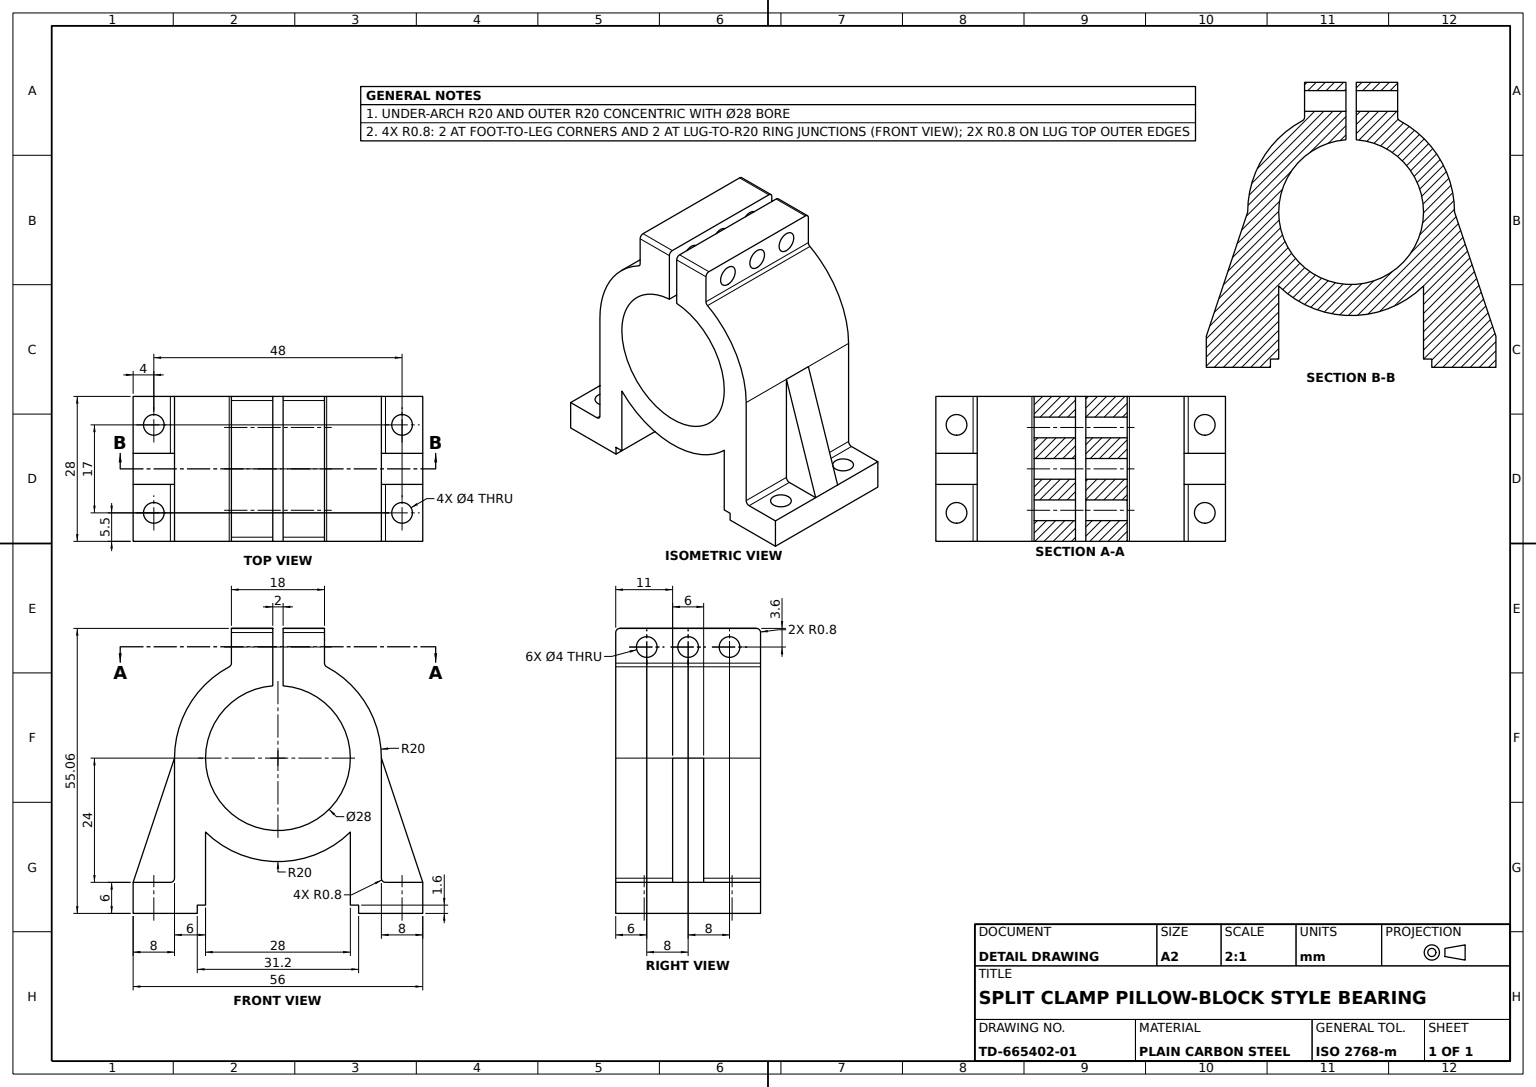
solid
v1 (-28,-24,-11)
v2 (-20.8,-24,-11)
e1 v1 v2 LINE
v3 (-28,-24,0)
e2 v1 v3 LINE
v4 (-20.8,-24,0)
e3 v4 v3 LINE
e4 v4 v2 LINE
v5 (-24,-24,-3.5)
v6 (-24,-24,-7.5)
e5 v5 v6 CIRCLE(AX(P(-24,-24,-5.5),D(0,1,0),D(0,0,1)),2)
e6 v6 v5 CIRCLE(AX(P(-24,-24,-5.5),D(0,1,0),D(0,0,1)),2)
face PLANE(AX(P(-20,-24,-28),D(0,1,0),D(0,0,1))) [-e1 e2 -e3 e4] [-e5 -e6]
v7 (-20,-23.2,-11)
v8 (-20,0,-11)
e7 v7 v8 LINE
e8 v8 v1 LINE
e9 v2 v7 CIRCLE(AX(P(-20.8,-23.2,-11),D(0,0,1),D(1,0,0)),0.8)
face PLANE(AX(P(0,-5,-11),D(0,0,1),D(1,0,0))) [e7 e8 e1 e9]
v9 (-1,23.460571,-22)
v10 (-1,19.460571,-22)
e10 v9 v10 CIRCLE(AX(P(-1,21.460571,-22),D(-1,0,0),D(0,0,1)),2)
v11 (-9,23.460571,-22)
e11 v11 v9 LINE
v12 (-9,19.460571,-22)
e12 v11 v12 CIRCLE(AX(P(-9,21.460571,-22),D(-1,0,0),D(0,0,1)),2)
e13 v12 v10 LINE
face CYL(AX(P(-19,21.460571,-22),D(1,0,0),D(0,1,0)),2) rev [-e10 -e11 e12 e13]
v13 (1,23.460571,-6)
v14 (1,19.460571,-6)
e14 v13 v14 CIRCLE(AX(P(1,21.460571,-6),D(1,0,0),D(0,0,-1)),2)
e15 v14 v13 CIRCLE(AX(P(1,21.460571,-6),D(1,0,0),D(0,0,-1)),2)
v15 (1,25.060571,-0.8)
v16 (1,25.060571,-27.2)
e16 v15 v16 LINE
v17 (1,24.260571,-28)
e17 v16 v17 CIRCLE(AX(P(1,24.260571,-27.2),D(-1,0,0),D(0,0,-1)),0.8)
v18 (1,13.96424,-28)
e18 v18 v17 LINE
v19 (1,13.96424,0)
e19 v19 v18 LINE
v20 (1,24.260571,0)
e20 v19 v20 LINE
e21 v20 v15 CIRCLE(AX(P(1,24.260571,-0.8),D(-1,0,0),D(0,0,-1)),0.8)
v21 (1,23.460571,-14)
v22 (1,19.460571,-14)
e22 v21 v22 CIRCLE(AX(P(1,21.460571,-14),D(1,0,0),D(0,0,-1)),2)
e23 v22 v21 CIRCLE(AX(P(1,21.460571,-14),D(1,0,0),D(0,0,-1)),2)
v23 (1,23.460571,-22)
v24 (1,19.460571,-22)
e24 v23 v24 CIRCLE(AX(P(1,21.460571,-22),D(1,0,0),D(0,0,-1)),2)
e25 v24 v23 CIRCLE(AX(P(1,21.460571,-22),D(1,0,0),D(0,0,-1)),2)
face PLANE(AX(P(1,11.884737,-28),D(1,0,0),D(0,0,-1))) rev [e14 e15] [e16 e17 -e18 -e19 e20 e21] [e22 e23] [e24 e25]
v25 (9,19.460571,-22)
e26 v24 v25 LINE
v26 (9,23.460571,-22)
e27 v23 v26 LINE
e28 v26 v25 CIRCLE(AX(P(9,21.460571,-22),D(1,0,0),D(0,1,0)),2)
face CYL(AX(P(-19,21.460571,-22),D(1,0,0),D(0,1,0)),2) rev [-e26 -e24 e27 e28]
v27 (-9.423077,17.641021,-28)
v28 (-9,18.346662,-28)
e29 v27 v28 CIRCLE(AX(P(-9.8,18.346662,-28),D(0,0,1),D(1,0,0)),0.8)
v29 (-9.423077,17.641021,0)
e30 v29 v27 LINE
v30 (-9,18.346662,0)
e31 v30 v29 CIRCLE(AX(P(-9.8,18.346662,0),D(0,0,-1),D(1,0,0)),0.8)
e32 v28 v30 LINE
face CYL(AX(P(-9.8,18.346662,-28),D(0,0,1),D(1,0,0)),0.8) rev [-e29 -e30 -e31 -e32]
v31 (-9,23.460571,-14)
v32 (-9,19.460571,-14)
e33 v31 v32 CIRCLE(AX(P(-9,21.460571,-14),D(-1,0,0),D(0,0,1)),2)
v33 (-1,19.460571,-14)
e34 v32 v33 LINE
v34 (-1,23.460571,-14)
e35 v34 v33 CIRCLE(AX(P(-1,21.460571,-14),D(-1,0,0),D(0,0,1)),2)
e36 v31 v34 LINE
face CYL(AX(P(-19,21.460571,-14),D(1,0,0),D(0,1,0)),2) rev [e33 e34 -e35 -e36]
v35 (20,0,-11)
v36 (28,-24,-11)
e37 v35 v36 LINE
v37 (28,-24,-17)
e38 v37 v36 LINE
v38 (20,0,-17)
e39 v38 v37 LINE
e40 v38 v35 LINE
face PLANE(AX(P(20,0,-14),D(-0.948683298,-0.316227766,0),D(0.316227766,-0.948683298,0))) rev [e37 -e38 -e39 e40]
v39 (-1,24.260571,-28)
v40 (-1,13.96424,-28)
e41 v39 v40 LINE
v41 (-1,25.060571,-27.2)
e42 v39 v41 CIRCLE(AX(P(-1,24.260571,-27.2),D(1,0,0),D(0,0,1)),0.8)
v42 (-1,25.060571,-0.8)
e43 v41 v42 LINE
v43 (-1,24.260571,0)
e44 v42 v43 CIRCLE(AX(P(-1,24.260571,-0.8),D(1,0,0),D(0,0,1)),0.8)
v44 (-1,13.96424,0)
e45 v43 v44 LINE
e46 v40 v44 LINE
e47 v10 v9 CIRCLE(AX(P(-1,21.460571,-22),D(-1,0,0),D(0,0,1)),2)
e48 v33 v34 CIRCLE(AX(P(-1,21.460571,-14),D(-1,0,0),D(0,0,1)),2)
v45 (-1,23.460571,-6)
v46 (-1,19.460571,-6)
e49 v45 v46 CIRCLE(AX(P(-1,21.460571,-6),D(-1,0,0),D(0,0,1)),2)
e50 v46 v45 CIRCLE(AX(P(-1,21.460571,-6),D(-1,0,0),D(0,0,1)),2)
face PLANE(AX(P(-1,11.884737,-28),D(-1,0,0),D(0,0,1))) rev [-e41 e42 e43 e44 e45 -e46] [e10 e47] [e35 e48] [e49 e50]
v47 (28,-30,-28)
v48 (28,-30,0)
e51 v47 v48 LINE
v49 (28,-24,-28)
e52 v47 v49 LINE
e53 v49 v37 LINE
v50 (28,-24,0)
e54 v36 v50 LINE
e55 v48 v50 LINE
face PLANE(AX(P(28,-24,-28),D(1,0,0),D(0,0,-1))) [-e51 e52 e53 e38 e54 -e55]
v51 (-14,0,0)
e56 v44 v51 CIRCLE(AX(P(0,0,0),D(0,0,1),D(1,0,0)),14)
v52 (-14,0,-28)
e57 v52 v51 LINE
e58 v40 v52 CIRCLE(AX(P(0,0,-28),D(0,0,1),D(1,0,0)),14)
face CYL(AX(P(0,0,-28),D(0,0,1),D(1,0,0)),14) rev [e56 -e57 -e58 e46]
v53 (24,-30,-24.5)
v54 (24,-24,-24.5)
e59 v53 v54 LINE
v55 (24,-30,-20.5)
e60 v53 v55 CIRCLE(AX(P(24,-30,-22.5),D(0,-1,0),D(0,0,-1)),2)
v56 (24,-24,-20.5)
e61 v55 v56 LINE
e62 v56 v54 CIRCLE(AX(P(24,-24,-22.5),D(0,1,0),D(0,0,1)),2)
face CYL(AX(P(24,-52,-22.5),D(0,1,0),D(0,0,1)),2) rev [-e59 e60 e61 e62]
v57 (9,25.060571,-27.2)
v58 (9,25.060571,-0.8)
e63 v57 v58 LINE
e64 v57 v16 LINE
e65 v15 v58 LINE
face PLANE(AX(P(-9,25.060571,-28),D(0,1,0),D(0,0,1))) [-e63 e64 -e16 e65]
v59 (-20,-23.2,-17)
v60 (-20,0,-17)
e66 v59 v60 LINE
v61 (-20,0,-28)
e67 v61 v60 LINE
v62 (-20,-23.2,-28)
e68 v61 v62 LINE
e69 v62 v59 LINE
face PLANE(AX(P(-20,0,-28),D(-1,0,0),D(0,0,1))) [e66 -e67 e68 e69]
v63 (24,-30,-7.5)
v64 (24,-24,-7.5)
e70 v63 v64 LINE
v65 (24,-24,-3.5)
e71 v64 v65 CIRCLE(AX(P(24,-24,-5.5),D(0,1,0),D(0,0,1)),2)
v66 (24,-30,-3.5)
e72 v66 v65 LINE
e73 v66 v63 CIRCLE(AX(P(24,-30,-5.5),D(0,-1,0),D(0,0,-1)),2)
face CYL(AX(P(24,-52,-5.5),D(0,1,0),D(0,0,1)),2) rev [e70 e71 -e72 e73]
v67 (20.8,-24,-17)
v68 (20,-23.2,-17)
e74 v67 v68 CIRCLE(AX(P(20.8,-23.2,-17),D(0,0,-1),D(1,0,0)),0.8)
e75 v38 v68 LINE
e76 v67 v37 LINE
face PLANE(AX(P(0,-5,-17),D(0,0,1),D(1,0,0))) rev [e74 -e75 e39 -e76]
e77 v27 v61 CIRCLE(AX(P(0,0,-28),D(0,0,1),D(1,0,0)),20)
v69 (-9,24.260571,-28)
e78 v69 v28 LINE
e79 v69 v39 LINE
v70 (14,0,-28)
e80 v52 v70 CIRCLE(AX(P(0,0,-28),D(0,0,1),D(1,0,0)),14)
e81 v70 v18 CIRCLE(AX(P(0,0,-28),D(0,0,1),D(1,0,0)),14)
v71 (9,24.260571,-28)
e82 v17 v71 LINE
v72 (9,18.346662,-28)
e83 v72 v71 LINE
v73 (9.423077,17.641021,-28)
e84 v72 v73 CIRCLE(AX(P(9.8,18.346662,-28),D(0,0,1),D(1,0,0)),0.8)
v74 (20,0,-28)
e85 v74 v73 CIRCLE(AX(P(0,0,-28),D(0,0,1),D(1,0,0)),20)
v75 (20,-23.2,-28)
e86 v75 v74 LINE
v76 (20.8,-24,-28)
e87 v75 v76 CIRCLE(AX(P(20.8,-23.2,-28),D(0,0,1),D(1,0,0)),0.8)
e88 v49 v76 LINE
v77 (15.6,-30,-28)
e89 v77 v47 LINE
v78 (15.6,-28.4,-28)
e90 v78 v77 LINE
v79 (14,-28.4,-28)
e91 v79 v78 LINE
v80 (14,-14.282857,-28)
e92 v80 v79 LINE
v81 (-14,-14.282857,-28)
e93 v81 v80 CIRCLE(AX(P(0,0,-28),D(0,0,1),D(1,0,0)),20)
v82 (-14,-28.4,-28)
e94 v82 v81 LINE
v83 (-15.6,-28.4,-28)
e95 v83 v82 LINE
v84 (-15.6,-30,-28)
e96 v84 v83 LINE
v85 (-28,-30,-28)
e97 v85 v84 LINE
v86 (-28,-24,-28)
e98 v86 v85 LINE
v87 (-20.8,-24,-28)
e99 v87 v86 LINE
e100 v87 v62 CIRCLE(AX(P(-20.8,-23.2,-28),D(0,0,1),D(1,0,0)),0.8)
face PLANE(AX(P(0,0,-28),D(0,0,1),D(1,0,0))) rev [-e68 -e77 e29 -e78 e79 e41 e58 e80 e81 e18 e82 -e83 e84 -e85 -e86 e87 -e88 -e52 -e89 -e90 -e91 -e92 -e93 -e94 -e95 -e96 -e97 -e98 -e99 e100]
v88 (9,24.260571,0)
e101 v58 v88 CIRCLE(AX(P(9,24.260571,-0.8),D(1,0,0),D(0,1,0)),0.8)
e102 v88 v20 LINE
face CYL(AX(P(0,24.260571,-0.8),D(-1,0,0),D(0,0,1)),0.8) [-e101 -e65 -e21 -e102]
v89 (14,-28.4,0)
v90 (15.6,-28.4,0)
e103 v89 v90 LINE
e104 v79 v89 LINE
e105 v78 v90 LINE
face PLANE(AX(P(14,-28.4,-28),D(0,-1,0),D(0,0,-1))) [-e103 -e104 e91 e105]
v91 (20,-23.2,-11)
e106 v35 v91 LINE
v92 (20,0,0)
e107 v35 v92 LINE
v93 (20,-23.2,0)
e108 v93 v92 LINE
e109 v93 v91 LINE
face PLANE(AX(P(20,0,-28),D(1,0,0),D(0,0,-1))) [-e106 e107 -e108 e109]
v94 (20.8,-24,-11)
e110 v94 v36 LINE
e111 v91 v94 CIRCLE(AX(P(20.8,-23.2,-11),D(0,0,1),D(1,0,0)),0.8)
face PLANE(AX(P(0,-5,-11),D(0,0,1),D(1,0,0))) [e110 -e37 e106 e111]
v95 (9,19.460571,-14)
e112 v22 v95 LINE
v96 (9,23.460571,-14)
e113 v95 v96 CIRCLE(AX(P(9,21.460571,-14),D(1,0,0),D(0,1,0)),2)
e114 v21 v96 LINE
face CYL(AX(P(-19,21.460571,-14),D(1,0,0),D(0,1,0)),2) rev [e112 e113 -e114 -e23]
v97 (-28,-24,-17)
e115 v60 v97 LINE
v98 (-20.8,-24,-17)
e116 v59 v98 CIRCLE(AX(P(-20.8,-23.2,-17),D(0,0,-1),D(1,0,0)),0.8)
e117 v97 v98 LINE
face PLANE(AX(P(0,-5,-17),D(0,0,1),D(1,0,0))) rev [-e115 -e66 e116 -e117]
v99 (9,19.460571,-6)
v100 (9,23.460571,-6)
e118 v99 v100 CIRCLE(AX(P(9,21.460571,-6),D(1,0,0),D(0,1,0)),2)
e119 v13 v100 LINE
e120 v14 v99 LINE
face CYL(AX(P(-19,21.460571,-6),D(1,0,0),D(0,1,0)),2) rev [e118 -e119 -e15 e120]
v101 (-24,-30,-20.5)
v102 (-24,-24,-20.5)
e121 v101 v102 LINE
v103 (-24,-24,-24.5)
e122 v102 v103 CIRCLE(AX(P(-24,-24,-22.5),D(0,1,0),D(0,0,1)),2)
v104 (-24,-30,-24.5)
e123 v104 v103 LINE
e124 v104 v101 CIRCLE(AX(P(-24,-30,-22.5),D(0,-1,0),D(0,0,-1)),2)
face CYL(AX(P(-24,-52,-22.5),D(0,1,0),D(0,0,1)),2) rev [e121 e122 -e123 e124]
v105 (14,-14.282857,0)
e125 v105 v89 LINE
e126 v80 v105 LINE
face PLANE(AX(P(14,-28.4,-28),D(-1,0,0),D(0,-1,0))) [e92 e104 -e125 -e126]
v106 (-20,-23.2,0)
e127 v7 v106 LINE
v107 (-20,0,0)
e128 v107 v106 LINE
e129 v8 v107 LINE
face PLANE(AX(P(-20,0,-28),D(-1,0,0),D(0,0,1))) [e127 -e128 -e129 -e7]
v108 (-9,19.460571,-6)
e130 v108 v46 LINE
v109 (-9,23.460571,-6)
e131 v108 v109 CIRCLE(AX(P(-9,21.460571,-6),D(-1,0,0),D(0,0,1)),2)
e132 v109 v45 LINE
face CYL(AX(P(-19,21.460571,-6),D(1,0,0),D(0,1,0)),2) rev [-e130 e131 e132 -e50]
e133 v25 v26 CIRCLE(AX(P(9,21.460571,-22),D(1,0,0),D(0,1,0)),2)
face CYL(AX(P(-19,21.460571,-22),D(1,0,0),D(0,1,0)),2) rev [e26 e133 -e27 -e25]
e134 v98 v87 LINE
face CYL(AX(P(-20.8,-23.2,-28),D(0,0,-1),D(-1,0,0)),0.8) rev [-e116 -e69 -e100 -e134]
v110 (-24,-30,-7.5)
e135 v110 v6 LINE
v111 (-24,-30,-3.5)
e136 v110 v111 CIRCLE(AX(P(-24,-30,-5.5),D(0,-1,0),D(0,0,-1)),2)
e137 v111 v5 LINE
face CYL(AX(P(-24,-52,-5.5),D(0,1,0),D(0,0,1)),2) rev [e5 -e135 e136 e137]
e138 v111 v110 CIRCLE(AX(P(-24,-30,-5.5),D(0,-1,0),D(0,0,-1)),2)
e139 v101 v104 CIRCLE(AX(P(-24,-30,-22.5),D(0,-1,0),D(0,0,-1)),2)
v112 (-15.6,-30,0)
e140 v84 v112 LINE
v113 (-28,-30,0)
e141 v113 v112 LINE
e142 v85 v113 LINE
face PLANE(AX(P(-28,-30,-28),D(0,-1,0),D(0,0,-1))) [-e136 -e138] [-e124 -e139] [e97 e140 -e141 -e142]
e143 v55 v53 CIRCLE(AX(P(24,-30,-22.5),D(0,-1,0),D(0,0,-1)),2)
e144 v54 v56 CIRCLE(AX(P(24,-24,-22.5),D(0,1,0),D(0,0,1)),2)
face CYL(AX(P(24,-52,-22.5),D(0,1,0),D(0,0,1)),2) rev [-e61 e143 e59 e144]
e145 v106 v4 CIRCLE(AX(P(-20.8,-23.2,0),D(0,0,-1),D(1,0,0)),0.8)
face CYL(AX(P(-20.8,-23.2,-28),D(0,0,-1),D(-1,0,0)),0.8) rev [-e9 -e4 -e145 -e127]
e146 v3 v113 LINE
e147 v97 v1 LINE
e148 v86 v97 LINE
face PLANE(AX(P(-28,-24,-28),D(-1,0,0),D(0,0,1))) [e142 -e146 -e2 -e147 -e148 e98]
v114 (-9,25.060571,-0.8)
e149 v114 v42 LINE
v115 (-9,24.260571,0)
e150 v115 v114 CIRCLE(AX(P(-9,24.260571,-0.8),D(-1,0,0),D(0,0,1)),0.8)
e151 v43 v115 LINE
face CYL(AX(P(0,24.260571,-0.8),D(-1,0,0),D(0,0,1)),0.8) [-e44 -e149 -e150 -e151]
e152 v100 v99 CIRCLE(AX(P(9,21.460571,-6),D(1,0,0),D(0,1,0)),2)
e153 v96 v95 CIRCLE(AX(P(9,21.460571,-14),D(1,0,0),D(0,1,0)),2)
v116 (9,18.346662,0)
e154 v116 v88 LINE
e155 v116 v72 LINE
e156 v71 v57 CIRCLE(AX(P(9,24.260571,-27.2),D(1,0,0),D(0,1,0)),0.8)
face PLANE(AX(P(9,17.860571,-28),D(1,0,0),D(0,1,0))) [-e152 -e118] [-e133 -e28] [-e113 -e153] [e63 e101 -e154 e155 e83 e156]
v117 (9.423077,17.641021,0)
e157 v117 v116 CIRCLE(AX(P(9.8,18.346662,0),D(0,0,-1),D(1,0,0)),0.8)
e158 v73 v117 LINE
face CYL(AX(P(9.8,18.346662,-28),D(0,0,1),D(1,0,0)),0.8) rev [-e84 -e155 -e157 -e158]
face CYL(AX(P(-24,-52,-5.5),D(0,1,0),D(0,0,1)),2) rev [e138 e135 e6 -e137]
v118 (-9,25.060571,-27.2)
e159 v41 v118 LINE
e160 v118 v114 LINE
face PLANE(AX(P(-9,25.060571,-28),D(0,1,0),D(0,0,1))) [e159 e160 e149 -e43]
e161 v60 v8 LINE
face PLANE(AX(P(-20,0,-14),D(-0.948683298,0.316227766,0),D(-0.316227766,-0.948683298,0))) [-e8 -e161 e115 e147]
e162 v109 v108 CIRCLE(AX(P(-9,21.460571,-6),D(-1,0,0),D(0,0,1)),2)
face CYL(AX(P(-19,21.460571,-6),D(1,0,0),D(0,1,0)),2) rev [-e132 e162 e130 -e49]
e163 v76 v67 LINE
face PLANE(AX(P(20,-24,-28),D(0,1,0),D(0,0,1))) [e88 e163 e76 -e53] [-e144 -e62]
face CYL(AX(P(-9,24.260571,-27.2),D(1,0,0),D(0,0,-1)),0.8) [-e17 -e64 -e156 -e82]
v119 (-14,-14.282857,0)
e164 v81 v119 LINE
v120 (-14,-28.4,0)
e165 v120 v119 LINE
e166 v82 v120 LINE
face PLANE(AX(P(-14,-28.4,-28),D(1,0,0),D(0,1,0))) [e94 e164 -e165 -e166]
v121 (20.8,-24,0)
e167 v94 v121 LINE
e168 v50 v121 LINE
e169 v65 v64 CIRCLE(AX(P(24,-24,-5.5),D(0,1,0),D(0,0,1)),2)
face PLANE(AX(P(20,-24,-28),D(0,1,0),D(0,0,1))) [e167 -e168 -e54 -e110] [-e71 -e169]
e170 v121 v93 CIRCLE(AX(P(20.8,-23.2,0),D(0,0,-1),D(1,0,0)),0.8)
face CYL(AX(P(20.8,-23.2,-28),D(0,0,-1),D(-1,0,0)),0.8) rev [-e111 -e109 -e170 -e167]
e171 v32 v31 CIRCLE(AX(P(-9,21.460571,-14),D(-1,0,0),D(0,0,1)),2)
face CYL(AX(P(-19,21.460571,-14),D(1,0,0),D(0,1,0)),2) rev [e171 e36 -e48 -e34]
e172 v74 v38 LINE
e173 v92 v117 CIRCLE(AX(P(0,0,0),D(0,0,1),D(1,0,0)),20)
face CYL(AX(P(0,0,-28),D(0,0,1),D(1,0,0)),20) [-e40 -e172 e85 e158 -e173 -e107]
e174 v63 v66 CIRCLE(AX(P(24,-30,-5.5),D(0,-1,0),D(0,0,-1)),2)
face CYL(AX(P(24,-52,-5.5),D(0,1,0),D(0,0,1)),2) rev [e174 e72 e169 -e70]
e175 v118 v69 CIRCLE(AX(P(-9,24.260571,-27.2),D(-1,0,0),D(0,0,1)),0.8)
face CYL(AX(P(-9,24.260571,-27.2),D(1,0,0),D(0,0,-1)),0.8) [-e175 -e159 -e42 -e79]
v122 (15.6,-30,0)
e176 v122 v48 LINE
e177 v77 v122 LINE
face PLANE(AX(P(28,-30,-28),D(0,-1,0),D(0,0,-1))) [-e73 -e174] [-e176 -e177 e89 e51] [-e60 -e143]
e178 v29 v107 CIRCLE(AX(P(0,0,0),D(0,0,1),D(1,0,0)),20)
face CYL(AX(P(0,0,-28),D(0,0,1),D(1,0,0)),20) [e129 -e178 e30 e77 e67 e161]
e179 v103 v102 CIRCLE(AX(P(-24,-24,-22.5),D(0,1,0),D(0,0,1)),2)
face PLANE(AX(P(-20,-24,-28),D(0,1,0),D(0,0,1))) [e99 e148 e117 e134] [-e122 -e179]
face CYL(AX(P(-19,21.460571,-6),D(1,0,0),D(0,1,0)),2) rev [e119 e152 -e120 -e14]
e180 v119 v105 CIRCLE(AX(P(0,0,0),D(0,0,1),D(1,0,0)),20)
face CYL(AX(P(0,0,-28),D(0,0,1),D(1,0,0)),20) [-e164 e93 e126 -e180]
face CYL(AX(P(-24,-52,-22.5),D(0,1,0),D(0,0,1)),2) rev [e179 -e121 e139 e123]
e181 v12 v11 CIRCLE(AX(P(-9,21.460571,-22),D(-1,0,0),D(0,0,1)),2)
face CYL(AX(P(-19,21.460571,-22),D(1,0,0),D(0,1,0)),2) rev [e11 -e47 -e13 e181]
e182 v90 v122 LINE
face PLANE(AX(P(15.6,-28.4,-28),D(-1,0,0),D(0,0,1))) [e90 e177 -e182 -e105]
face CYL(AX(P(-19,21.460571,-14),D(1,0,0),D(0,1,0)),2) rev [e153 -e112 -e22 e114]
e183 v115 v30 LINE
face PLANE(AX(P(-9,17.860571,-28),D(-1,0,0),D(0,0,1))) [e78 e32 -e183 e150 -e160 e175] [-e181 -e12] [-e162 -e131] [-e171 -e33]
e184 v68 v75 LINE
face PLANE(AX(P(20,0,-28),D(1,0,0),D(0,0,-1))) [e86 e172 e75 e184]
v123 (-15.6,-28.4,0)
e185 v123 v120 LINE
e186 v83 v123 LINE
face PLANE(AX(P(-14,-28.4,-28),D(0,-1,0),D(1,0,0))) [e95 e166 -e185 -e186]
v124 (14,0,0)
e187 v51 v124 CIRCLE(AX(P(0,0,0),D(0,0,1),D(1,0,0)),14)
e188 v70 v124 LINE
face CYL(AX(P(0,0,-28),D(0,0,1),D(1,0,0)),14) rev [e187 -e188 -e80 e57]
e189 v124 v19 CIRCLE(AX(P(0,0,0),D(0,0,1),D(1,0,0)),14)
e190 v112 v123 LINE
face PLANE(AX(P(0,0,0),D(0,0,1),D(1,0,0))) [e154 e102 -e20 -e189 -e187 -e56 -e45 e151 e183 e31 e178 e128 e145 e3 e146 e141 e190 e185 e165 e180 e125 e103 e182 e176 e55 e168 e170 e108 e173 e157]
face CYL(AX(P(20.8,-23.2,-28),D(0,0,-1),D(-1,0,0)),0.8) rev [-e184 -e74 -e163 -e87]
face CYL(AX(P(0,0,-28),D(0,0,1),D(1,0,0)),14) rev [e19 -e81 e188 e189]
face PLANE(AX(P(-15.6,-28.4,-28),D(1,0,0),D(0,0,-1))) [-e140 e96 e186 -e190]
